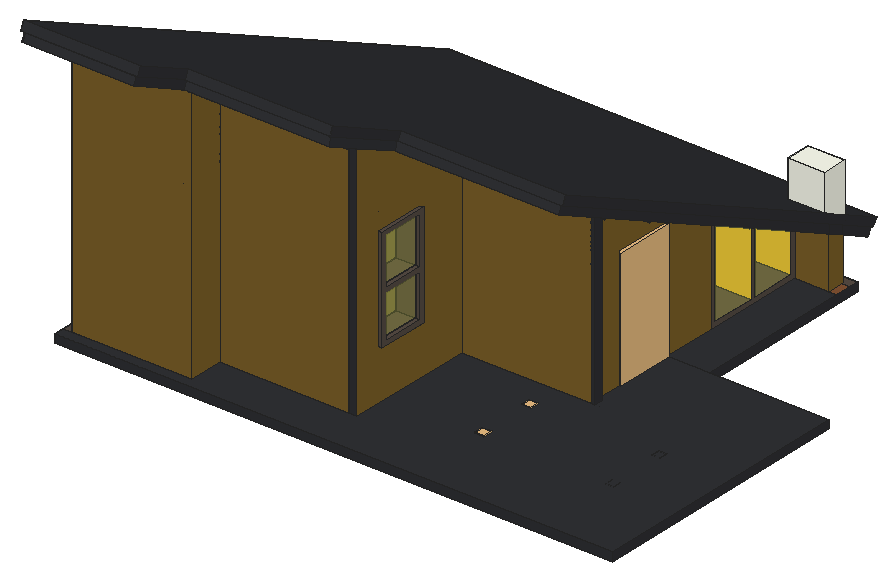
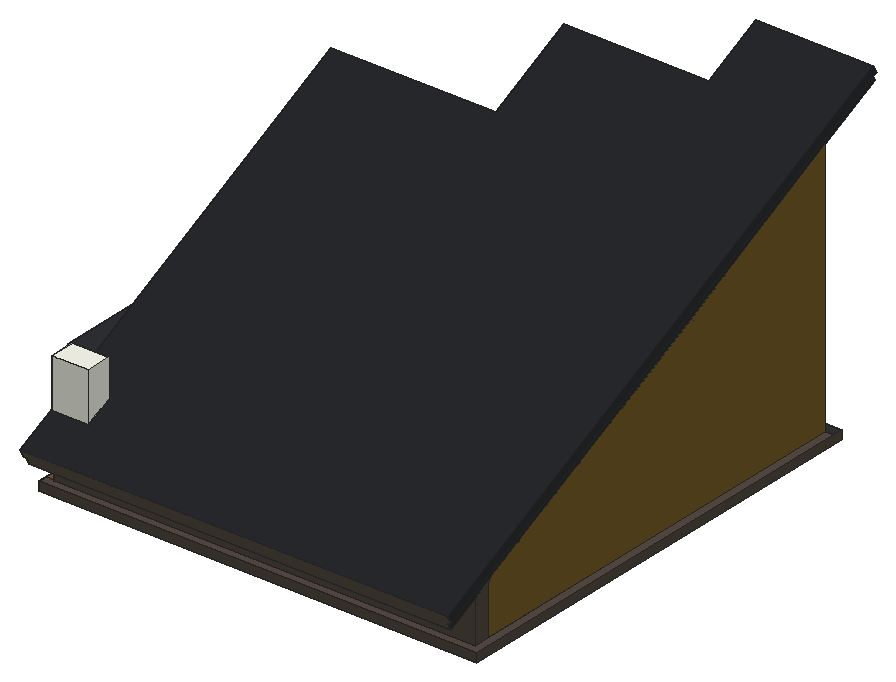
# SketchUp Ruby script. Lengths in inches.
U = 1.inch
M = Sketchup.active_model
def pt(a) = Geom::Point3d.new(a.map { |v| v * U })
def face(e, loops, mat)
  f = e.add_face(loops[0].map { |a| pt(a) })
  loops[1..].each { |l| e.add_face(l.map { |a| pt(a) }).erase! }
  f.material = f.back_material = mat if mat
  f
end
# faces: each face lists its corners as indices into pts; further lists are holes
def faces(e, pts, list, mat = nil) = list.each { |f| face(e, (f[0].is_a?(Array) ? f : [f]).map { |l| l.map { |i| pts[i] } }, mat) }
# xy, xz, yz: faces in a plane at the given z, y or x. An outline is a flat list of corners, or four numbers for a rectangle; further outlines are holes
def ring(l) = l.size == 4 ? [[l[0], l[1]], [l[2], l[1]], [l[2], l[3]], [l[0], l[3]]] : l.each_slice(2).to_a
def flat(e, list, mat, &to3) = list.each { |f| face(e, (f[0].is_a?(Array) ? f : [f]).map { |l| ring(l).map { |u, v| to3.(u, v) } }, mat) }
def xy(e, z, list, mat = nil) = flat(e, list, mat) { |x, y| [x, y, z] }
def xz(e, y, list, mat = nil) = flat(e, list, mat) { |x, z| [x, y, z] }
def yz(e, x, list, mat = nil) = flat(e, list, mat) { |y, z| [x, y, z] }
def lines(e, pts, list) = list.each { |a, b| e.add_line(pt(pts[a]), pt(pts[b])) }
# prism: a flat outline (further loops are holes) pulled along v
def prism(e, loops, v, mat = nil)
  f = face(e, loops, mat); d = Geom::Vector3d.new(v.map { |x| x * U })
  f.pushpull(f.normal.samedirection?(d) ? d.length : -d.length)
end
def box(e, o, s, mat = nil) = prism(e, [[o, [o[0] + s[0], o[1], o[2]], [o[0] + s[0], o[1] + s[1], o[2]], [o[0], o[1] + s[1], o[2]]]], [0, 0, s[2]], mat)
def at(x, y, z, deg = 0) = Geom::Transformation.translation(pt([x, y, z])) * Geom::Transformation.rotation(ORIGIN, Z_AXIS, deg.degrees)
def axes(o, x, y, z) = Geom::Transformation.new([*x, 0, *y, 0, *z, 0, *pt(o).to_a, 1])
def part(name) = M.definitions.add(name)
# library, detail: a bought-in or finely detailed component or shape, given as its bounding box
def library(name, o, s) = part(name).tap { |d| box(d.entities, o, s) }
def detail(e, o, s) = box(e.add_group.entities, o, s)
def put(e, d, t, mat = nil) = e.add_instance(d, t).tap { |i| i.material = mat if mat }
def group(e, t, mat = nil) = e.add_group.tap { |g| g.transformation = t; g.material = mat if mat }.entities
root = M.entities
M.materials.add("Asphalt_02_1K").color = [86, 76, 68]
M.materials.add("Concrete_04_1K").color = [254, 255, 241]
M.materials.add("D04_Dandelion_Burst").color = [255, 204, 50]
M.materials.add("Glass_Basic_01").color = [253, 255, 84]
M.materials["Glass_Basic_01"].alpha = 0.25
M.materials.add("Plywood_01_1K").color = [130, 82, 50]
M.materials.add("Plywood_01_1K1").color = [125, 97, 41]
M.materials.add("ThomThom - Buttons1").color = [48, 49, 53]
M.materials.add("ThomThom - Buttons2").color = [40, 40, 43]
c1 = library("Sphere Light\#2",[-3.27,-3.27,-3.27],[6.54,6.54,6.54])
c2 = library("Sphere Light\#3",[-3.12,-3.12,-3.12],[6.24,6.24,6.24])
c3 = library("Sphere Light",[-2.87,-2.87,-2.87],[5.74,5.74,5.74])
c4 = library("Sphere Light\#1",[-2.75,-2.75,-2.75],[5.5,5.5,5.5])
c5 = library("porta+4",[0.2,-5.42,1.33],[46.55,4.72,83.21])
c6 = library("Sphere Light\#4",[-2.75,-2.75,-2.75],[5.5,5.5,5.5])
c7 = library("Sphere Light\#5",[-3.11,-3.11,-3.11],[6.22,6.22,6.22])
c8 = library("Sphere Light\#6",[-2.79,-2.79,-2.79],[5.58,5.58,5.58])
c9 = library("Sphere Light\#7",[-3.09,-3.09,-3.09],[6.18,6.18,6.18])
c10 = library("Sphere Light\#8",[-2.99,-2.99,-2.99],[5.98,5.98,5.98])
xy(root,120,[[[24,80.18,24,398.18,330,398.18,330,269.18,413,269.18,413,80.18],[262.73,128.19,377,192.97],[377,116.19,389,128.19]],[[262.73,128.19,377,192.97],[274.73,137.19,275.51,137.29,276.23,137.59,276.85,138.07,277.33,138.69,277.63,139.42,277.73,140.19,362,140.19,362.1,139.42,362.4,138.69,362.88,138.07,363.5,137.59,364.22,137.29,365,137.19,365.78,137.29,366.5,137.59,367.12,138.07,367.6,138.69,367.9,139.42,368,140.19,367.9,140.97,367.6,141.69,367.12,142.3125,366.5,142.79,365.78,143.09,365,143.19,365,178,365.43,178,366.19,178.21,366.86,178.62,367.4,179.18,367.79,179.86,367.98,180.62,367.97,181.4,367.76,182.16,367.36,182.83,366.79,183.375,366.11,183.76,365.35,183.95,364.57,183.9375,363.81,183.73,363.14,183.33,362.6,182.76,362.21,182.08,362.02,181.32,362.03,180.97,277.73,180.97,277.63,181.75,277.33,182.47,276.85,183.09,276.23,183.57,275.51,183.87,274.73,183.97,273.96,183.87,273.23,183.57,272.61,183.09,272.14,182.47,271.84,181.75,271.73,180.97,271.84,180.19,272.14,179.47,272.61,178.85,273.23,178.37,273.96,178.07,274.73,177.97,274.73,143.19,273.96,143.09,273.23,142.79,272.61,142.3125,272.14,141.69,271.84,140.97,271.73,140.19,271.84,139.42,272.14,138.69,272.61,138.07,273.23,137.59,273.96,137.29]],[277.73,140.19,277.63,140.97,277.33,141.69,276.85,142.3125,276.23,142.79,275.51,143.09,274.73,143.19,274.73,177.97,275.51,178.07,276.23,178.37,276.85,178.85,277.33,179.47,277.63,180.19,277.73,180.97,362.03,180.97,362.03,180.54,362.24,179.79,362.64,179.11,363.21,178.57,363.89,178.18,364.65,177.99,365,178,365,143.19,364.22,143.09,363.5,142.79,362.88,142.3125,362.4,141.69,362.1,140.97,362,140.19]],"ThomThom - Buttons2")
xy(root,123,[[274.73,137.19,273.96,137.29,273.23,137.59,272.61,138.07,272.14,138.69,271.84,139.42,271.73,140.19,271.84,140.97,272.14,141.69,272.61,142.3125,273.23,142.79,273.96,143.09,274.73,143.19,275.51,143.09,276.23,142.79,276.85,142.3125,277.33,141.69,277.63,140.97,277.73,140.19,277.63,139.42,277.33,138.69,276.85,138.07,276.23,137.59,275.51,137.29],[365,137.19,364.22,137.29,363.5,137.59,362.88,138.07,362.4,138.69,362.1,139.42,362,140.19,362.1,140.97,362.4,141.69,362.88,142.3125,363.5,142.79,364.22,143.09,365,143.19,365.78,143.09,366.5,142.79,367.12,142.3125,367.6,141.69,367.9,140.97,368,140.19,367.9,139.42,367.6,138.69,367.12,138.07,366.5,137.59,365.78,137.29],[274.73,177.97,273.96,178.07,273.23,178.37,272.61,178.85,272.14,179.47,271.84,180.19,271.73,180.97,271.84,181.75,272.14,182.47,272.61,183.09,273.23,183.57,273.96,183.87,274.73,183.97,275.51,183.87,276.23,183.57,276.85,183.09,277.33,182.47,277.63,181.75,277.73,180.97,277.63,180.19,277.33,179.47,276.85,178.85,276.23,178.37,275.51,178.07],[364.65,177.99,363.89,178.18,363.21,178.57,362.64,179.11,362.24,179.79,362.03,180.54,362.03,180.97,362.02,181.32,362.21,182.08,362.6,182.76,363.14,183.33,363.81,183.73,364.57,183.9375,365.35,183.95,366.11,183.76,366.79,183.375,367.36,182.83,367.76,182.16,367.97,181.4,367.98,180.62,367.79,179.86,367.4,179.18,366.86,178.62,366.19,178.21,365.43,178,365,178]],"ThomThom - Buttons2")
xy(root,126,[[24,87.33,30,87.33,30,392.18,330,392.18,330,398.18,24,398.18],[36,93.33,108,93.33,108,136.18,196.36,136.18,196.36,202.18,36,202.18],[204,111.33,210,130.18],[114,117.33,204,130.18],[114,130.18,196.36,136.18],
  [196.36,130.18,204,136.18],[204,130.18,210,130.18,210,202.18,303,202.18,303,208.18,204,208.18,204,202.18,196.36,202.18,196.36,136.18,204,136.18],[30,202.18,36,380.18],[36,202.18,204,208.18],[36,208.18,108,380.18],
  [108,208.18,114,380.18],[114,208.18,204,380.18],[204,208.18,210,380.18],[210,208.18,294,380.18],[294,208.18,300,227.18],
  [294,269.18,300,380.18]],"Asphalt_02_1K")
xy(root,126,[[324,380.18,330,392.18]],"Plywood_01_1K")
xy(root,126,[[24,80.18,413,80.18,413,269.18,294,269.18,294,227.18,300,227.18,300,208.18,303,208.18,303,202.18,210,202.18,210,111.33,114,111.33,114,87.33,24,87.33],[300,269.18,330,380.18]],"ThomThom - Buttons1")
xy(root,129,[[267.06,311.18,300,342.68],[267.06,345.68,300,377.18]],"Asphalt_02_1K")
xy(root,162,[[210,129.33,213,165.33]],"Asphalt_02_1K")
xy(root,165,[[196.36,132.33,210,162.33],[210,132.33,213,162.33]],"Asphalt_02_1K")
xy(root,172.02,[[300,374.18,319.02,380.18],[319.02,374.18,324,380.18]],"Concrete_04_1K")
xy(root,195,[[196.36,132.33,210,162.33],[210,132.33,213,162.33]],"Asphalt_02_1K")
xy(root,198,[[196.36,132.33,210,162.33],[210,132.33,213,162.33]],"Asphalt_02_1K")
xy(root,203.52,[[300,374.18,325.7,392.18]],"Concrete_04_1K")
xy(root,210,[[294,227.18,300,269.18]],"Plywood_01_1K")
xy(root,231,[[196.36,132.33,210,162.33],[210,132.33,213,162.33]],"Asphalt_02_1K")
xy(root,234,[[210,129.33,213,165.33]],"Asphalt_02_1K")
xy(root,246,[[36,93.33,108,202.18],[108,130.18,114,136.18],[108,136.18,196.36,202.18],[196.36,136.18,204,202.18],[108,202.18,114,208.18],
  [114,202.18,196.36,208.18],[196.36,202.18,204,208.18],[204,202.18,210,208.18],[210,202.18,303,208.18]],"Asphalt_02_1K")
xy(root,290.37,[[114,111.33,204,117.33]],"Asphalt_02_1K")
xz(root,80.18,[[24,120,413,126]],"ThomThom - Buttons1")
xz(root,87.33,[[30,126,114,305.02]],"Plywood_01_1K1")
xz(root,93.33,[[36,126,108,246]],"Asphalt_02_1K")
xz(root,111.33,[[114,126,204,290.37]],"Plywood_01_1K1")
xz(root,111.33,[[204,126,210,293.3],[114,290.37,204,293.3]],"ThomThom - Buttons1")
xz(root,117.33,[[114,126,204,290.37]],"Asphalt_02_1K")
xz(root,129.33,[[210,162,213,234]],"Asphalt_02_1K")
xz(root,130.18,[[196.36,126,204,246],[196.36,246,204,284.09]],"Asphalt_02_1K")
xz(root,132.33,[[196.36,165,210,195],[210,165,213,195],[196.36,198,210,231],[210,198,213,231]],"Asphalt_02_1K")
xz(root,136.18,[[108,126,114,246]],"Asphalt_02_1K")
xz(root,162.33,[[196.36,165,210,195],[210,165,213,195],[196.36,198,210,231],[210,198,213,231]],"Asphalt_02_1K")
xz(root,165.33,[[210,162,213,234]],"Asphalt_02_1K")
xz(root,178,[[365,120,365.43,123]],"ThomThom - Buttons2")
xz(root,202.18,[[36,126,196.36,246],[196.36,126,204,246]],"Asphalt_02_1K")
xz(root,202.18,[[210,126,300,246]],"Plywood_01_1K1")
xz(root,202.18,[[300,126,303,246],[210,246,303,248.93]],"ThomThom - Buttons1")
xz(root,208.18,[[36,126,108,246],[108,126,114,246],[114,126,204,246],[204,126,210,246],[210,126,294,246],
  [294,126,300,246]],"Asphalt_02_1K")
xz(root,208.18,[[300,126,303,246]],"ThomThom - Buttons1")
xz(root,227.18,[[294,126,300,210]],"Plywood_01_1K")
xz(root,269.18,[[294,126,300,210]],"Plywood_01_1K")
xz(root,269.18,[[330,120,413,126]],"ThomThom - Buttons1")
xz(root,311.18,[[267.06,129,300,192.36]],"D04_Dandelion_Burst")
xz(root,342.68,[[267.06,129,300,176.98]],"D04_Dandelion_Burst")
xz(root,345.68,[[267.06,129,300,175.51]],"D04_Dandelion_Burst")
xz(root,374.18,[[300,178.28,325.7,203.52]],"Concrete_04_1K")
xz(root,377.18,[[267.06,129,300,160.125]],"D04_Dandelion_Burst")
xz(root,380.18,[[30,126,36,162],[36,126,108,162],[108,126,114,162],[114,126,204,162],[204,126,210,162],
  [210,126,294,162],[294,126,300,162],[300,162,324,172.02]],"Asphalt_02_1K")
xz(root,380.18,[[300,126,324,162]],"Plywood_01_1K1")
xz(root,392.18,[[30,126,324,156.14]],"Asphalt_02_1K")
xz(root,392.18,[[300,166.16,325.7,203.52]],"Concrete_04_1K")
xz(root,398.18,[[24,120,330,126]],"Asphalt_02_1K")
yz(root,24,[[80.18,120,398.18,126]],"Asphalt_02_1K")
yz(root,28,[[416.48,150.95,46.83,331.48,45.03,332.35,47.67,337.75,419.11,156.34]],"ThomThom - Buttons1")
yz(root,30,[[380.18,126,380.18,162,392.18,156.14,392.18,126]],"Asphalt_02_1K")
yz(root,30,[[87.33,126,87.33,305.02,208.18,246,380.18,162,380.18,126]],"Plywood_01_1K1")
yz(root,30,[[413.84,145.5625,392.18,156.14,380.18,162,208.18,246,87.33,305.02,44.2,326.09,46.83,331.48,416.48,150.95]],"ThomThom - Buttons1")
yz(root,36,[[93.33,126,202.18,246],[208.18,126,380.18,126,380.18,162,208.18,246]],"Asphalt_02_1K")
yz(root,108,[[93.33,126,116.18,246],[116.18,126,130.18,246],[130.18,126,136.18,246],[208.18,126,208.18,246,380.18,162,380.18,126]],"Asphalt_02_1K")
yz(root,108,[[87.33,305.02,89.96,310.41,80.27,315.15,46.83,331.48,44.2,326.09]],"ThomThom - Buttons1")
yz(root,110,[[85.96,312.37,88.59,317.76,47.67,337.75,45.03,332.35,80.27,315.15]],"ThomThom - Buttons1")
yz(root,114,[[117.33,126,130.18,246],[130.18,126,136.18,246],[208.18,126,380.18,126,380.18,162,208.18,246],[111.33,246,117.33,290.37],[117.33,246,130.18,246,130.18,284.09,117.33,290.37],
  [111.33,290.37,117.33,290.37,111.33,293.3]],"Asphalt_02_1K")
yz(root,114,[[87.33,126,111.33,126,111.33,293.3,87.33,305.02]],"Plywood_01_1K1")
yz(root,196.36,[[[130.18,126,202.18,246],[132.33,198,162.33,231],[132.33,165,162.33,195]],[130.18,246,130.18,284.09,208.18,246]],"Asphalt_02_1K")
yz(root,196.36,[[132.33,165,162.33,195],[132.33,198,162.33,231]],"Glass_Basic_01")
yz(root,204,[[111.33,126,117.33,290.37],[117.33,126,130.18,246],[202.18,126,208.18,246],[208.18,126,208.18,246,380.18,162,380.18,126],[111.33,290.37,111.33,293.3,117.33,290.37]],"Asphalt_02_1K")
yz(root,210,[[208.18,126,380.18,126,380.18,162,208.18,246],[202.18,246,208.18,246,202.18,248.93]],"Asphalt_02_1K")
yz(root,210,[[132.33,165,162.33,195],[132.33,198,162.33,231]],"Glass_Basic_01")
yz(root,210,[[[111.33,126,202.18,126,202.18,248.93,144.52,277.09,111.33,293.3],[129.33,162,165.33,234]]],"Plywood_01_1K1")
yz(root,210.9,[[145.36,283.36,147.99,288.75,88.59,317.76,85.96,312.37]],"ThomThom - Buttons1")
yz(root,213,[[[129.33,162,165.33,234],[132.33,198,162.33,231],[132.33,165,162.33,195]]],"Asphalt_02_1K")
yz(root,267.06,[[311.18,129,342.68,129,342.68,176.98,311.18,192.36],[345.68,129,377.18,129,377.18,160.125,345.68,175.51]],"D04_Dandelion_Burst")
yz(root,294,[[227.18,126,269.18,210]],"Plywood_01_1K")
yz(root,300,[[[308.18,126,380.18,126,380.18,162,308.18,197.16],[311.18,129,311.18,192.36,342.68,176.98,342.68,129],[345.68,129,345.68,175.51,377.18,160.125,377.18,129]],[392.18,156.14,392.18,162,380.18,162]],"Asphalt_02_1K")
yz(root,300,[[392.18,166.16,380.18,172.02,381.5,174.71,392.18,169.49],[392.18,169.49,381.5,174.71,380.18,172.02,374.18,172.02,374.18,203.52,392.18,203.52]],"Concrete_04_1K")
yz(root,300,[[311.18,129,342.68,129,342.68,176.98,311.18,192.36],[345.68,129,377.18,129,377.18,160.125,345.68,175.51]],"Glass_Basic_01")
yz(root,300,[[208.18,126,227.18,126,227.18,210,269.18,210,269.18,126,308.18,126,308.18,197.16,208.18,246]],"Plywood_01_1K1")
yz(root,303,[[202.18,126,208.18,246],[202.18,246,208.18,246,202.18,248.93]],"ThomThom - Buttons1")
yz(root,324,[[380.18,126,392.18,126,392.18,156.14,380.18,162]],"Plywood_01_1K1")
yz(root,324,[[413.84,145.5625,416.48,150.95,392.18,162.82,392.18,156.14],[392.18,156.14,392.18,162.82,380.18,168.68,380.18,162],[380.18,162,380.18,168.68,147.15,282.48,144.52,277.09]],"ThomThom - Buttons1")
yz(root,325.7,[[392.18,166.16,392.18,203.52,374.18,203.52,374.18,178.28,375.5,177.64,381.5,174.71,380.18,172.02]],"Concrete_04_1K")
yz(root,326,[[416.48,150.95,419.11,156.34,381.5,174.71,375.5,177.64,374.18,178.28,147.99,288.75,145.36,283.36]],"ThomThom - Buttons1")
yz(root,330,[[269.18,120,398.18,126]],"ThomThom - Buttons1")
yz(root,362.03,[[180.54,120,180.97,123]],"ThomThom - Buttons2")
yz(root,413,[[80.18,120,269.18,126]],"ThomThom - Buttons1")
p = [[305.66,263.57,36.875],[305.66,233.28,36.875],[305.71,233.28,31.86],[305.71,263.57,31.86],[305.33,263.57,66.67],[305.33,233.28,66.67],
  [305.4,233.28,59.8],[305.4,263.57,59.8],[274.73,137.19,120],[273.96,137.29,120],[273.96,137.29,123],[274.73,137.19,123],
  [275.51,137.29,120],[275.51,137.29,123],[365,137.19,120],[364.22,137.29,120],[364.22,137.29,123],[365,137.19,123],
  [365.78,137.29,120],[365.78,137.29,123],[273.23,137.59,120],[273.23,137.59,123],[276.23,137.59,120],[276.23,137.59,123],
  [363.5,137.59,120],[363.5,137.59,123],[366.5,137.59,120],[366.5,137.59,123],[272.61,138.07,120],[272.61,138.07,123],
  [276.85,138.07,120],[276.85,138.07,123],[362.88,138.07,120],[362.88,138.07,123],[367.12,138.07,120],[367.12,138.07,123],
  [272.14,138.69,120],[272.14,138.69,123],[277.33,138.69,120],[277.33,138.69,123],[362.4,138.69,120],[362.4,138.69,123],
  [367.6,138.69,120],[367.6,138.69,123],[271.84,139.42,120],[271.84,139.42,123],[277.63,139.42,120],[277.63,139.42,123],
  [362.1,139.42,120],[362.1,139.42,123],[367.9,139.42,120],[367.9,139.42,123],[271.73,140.19,120],[271.73,140.19,123],
  [277.73,140.19,120],[277.73,140.19,123],[362,140.19,120],[362,140.19,123],[368,140.19,120],[368,140.19,123],
  [271.84,140.97,120],[271.84,140.97,123],[277.63,140.97,120],[277.63,140.97,123],[362.1,140.97,120],[362.1,140.97,123],
  [367.9,140.97,120],[367.9,140.97,123],[272.14,141.69,120],[272.14,141.69,123],[277.33,141.69,120],[277.33,141.69,123],
  [362.4,141.69,120],[362.4,141.69,123],[367.6,141.69,120],[367.6,141.69,123],[272.61,142.3125,120],[272.61,142.3125,123],
  [276.85,142.3125,120],[276.85,142.3125,123],[362.88,142.3125,120],[362.88,142.3125,123],[367.12,142.3125,120],[367.12,142.3125,123],
  [273.23,142.79,120],[273.23,142.79,123],[276.23,142.79,120],[276.23,142.79,123],[363.5,142.79,120],[363.5,142.79,123],
  [366.5,142.79,120],[366.5,142.79,123],[273.96,143.09,120],[273.96,143.09,123],[275.51,143.09,120],[275.51,143.09,123],
  [364.22,143.09,120],[364.22,143.09,123],[365.78,143.09,120],[365.78,143.09,123],[274.73,143.19,120],[274.73,143.19,123],
  [365,143.19,120],[365,143.19,123],[274.73,177.97,120],[273.96,178.07,120],[273.96,178.07,123],[274.73,177.97,123],
  [275.51,178.07,120],[275.51,178.07,123],[364.65,177.99,120],[363.89,178.18,120],[363.89,178.18,123],[364.65,177.99,123],
  [365,178,120],[365,178,123],[366.19,178.21,120],[365.43,178,120],[365.43,178,123],[366.19,178.21,123],
  [273.23,178.37,120],[273.23,178.37,123],[276.23,178.37,120],[276.23,178.37,123],[363.21,178.57,120],[363.21,178.57,123],
  [366.86,178.62,120],[366.86,178.62,123],[272.61,178.85,120],[272.61,178.85,123],[276.85,178.85,120],[276.85,178.85,123],
  [362.64,179.11,120],[362.64,179.11,123],[367.4,179.18,120],[367.4,179.18,123],[272.14,179.47,120],[272.14,179.47,123],
  [277.33,179.47,120],[277.33,179.47,123],[362.24,179.79,120],[362.24,179.79,123],[367.79,179.86,120],[367.79,179.86,123],
  [271.84,180.19,120],[271.84,180.19,123],[277.63,180.19,120],[277.63,180.19,123],[362.03,180.54,120],[362.03,180.54,123],
  [367.98,180.62,120],[367.98,180.62,123],[271.73,180.97,120],[271.73,180.97,123],[277.73,180.97,120],[277.73,180.97,123],
  [367.97,181.4,120],[367.97,181.4,123],[271.84,181.75,120],[271.84,181.75,123],[277.63,181.75,120],[277.63,181.75,123],
  [362.03,180.97,120],[362.02,181.32,120],[362.02,181.32,123],[362.03,180.97,123],[362.21,182.08,120],[362.21,182.08,123],
  [367.76,182.16,120],[367.76,182.16,123],[272.14,182.47,120],[272.14,182.47,123],[277.33,182.47,120],[277.33,182.47,123],
  [362.6,182.76,120],[362.6,182.76,123],[367.36,182.83,120],[367.36,182.83,123],[272.61,183.09,120],[272.61,183.09,123],
  [276.85,183.09,120],[276.85,183.09,123],[363.14,183.33,120],[363.14,183.33,123],[366.79,183.375,120],[366.79,183.375,123],
  [273.23,183.57,120],[273.23,183.57,123],[276.23,183.57,120],[276.23,183.57,123],[363.81,183.73,120],[363.81,183.73,123],
  [366.11,183.76,120],[366.11,183.76,123],[273.96,183.87,120],[273.96,183.87,123],[275.51,183.87,120],[275.51,183.87,123],
  [364.57,183.9375,120],[364.57,183.9375,123],[365.35,183.95,120],[365.35,183.95,123],[274.73,183.97,120],[274.73,183.97,123],
  [30,413.84,145.5625],[324,413.84,145.5625],[324,392.18,156.14],[300,392.18,156.14],[294,392.18,156.14],[210,392.18,156.14],
  [204,392.18,156.14],[114,392.18,156.14],[108,392.18,156.14],[36,392.18,156.14],[30,392.18,156.14],[324,416.48,150.95],
  [30,416.48,150.95],[28,416.48,150.95],[28,419.11,156.34],[326,419.11,156.34],[326,416.48,150.95],[299.65,266,157.55],
  [299.65,230.78,157.55],[299.73,230.78,150.125],[299.73,266,150.125],[30,46.83,331.48],[28,46.83,331.48],[324,147.15,282.48],
  [324,380.18,168.68],[324,392.18,162.82],[326,145.36,283.36],[324,145.36,283.36],[30,380.18,162],[36,380.18,162],
  [108,380.18,162],[114,380.18,162],[204,380.18,162],[210,380.18,162],[294,380.18,162],[300,380.18,162],
  [324,380.18,162],[325.7,375.5,177.64],[325.7,381.5,174.71],[326,381.5,174.71],[28,47.67,337.75],[110,47.67,337.75],
  [110,88.59,317.76],[210.9,88.59,317.76],[210.9,147.99,288.75],[326,147.99,288.75],[326,374.18,178.28],[325.7,374.18,178.28],
  [300,377.18,160.125],[300,345.68,175.51],[267.06,345.68,175.51],[267.06,377.18,160.125],[300,308.18,197.16],[324,144.52,277.09],
  [210,144.52,277.09],[210,202.18,248.93],[303,202.18,248.93],[303,208.18,246],[300,208.18,246],[313.75,361.64,171.06],
  [312.98,361.75,171],[312.2,361.67,171.04],[311.47,361.42,171.16],[310.84,361,171.37],[310.34,360.46,171.63],[310.03,359.8125,171.95],
  [309.91,359.12,172.29],[309.99,358.42,172.63],[310.27,357.76,172.95],[310.73,357.19,173.23],[311.34,356.75,173.44],[312.06,356.47,173.58],
  [312.83,356.36,173.64],[313.61,356.43,173.6],[314.34,356.69,173.48],[314.97,357.1,173.27],[315.47,357.65,173.01],[315.78,358.29,172.69],
  [315.9,358.99,172.35],[315.82,359.6875,172.01],[315.54,360.34,171.6875],[315.08,360.91,171.41],[314.47,361.35,171.2],[316.81,283.77,209.08],
  [316.72,284.47,208.74],[316.44,285.13,208.42],[315.98,285.7,208.14],[315.37,286.14,207.93],[314.65,286.43,207.79],[313.88,286.53,207.74],
  [313.1,286.46,207.77],[312.37,286.21,207.9],[311.74,285.79,208.1],[311.25,285.24,208.37],[310.93,284.6,208.68],[310.81,283.91,209.02],
  [310.89,283.21,209.36],[311.17,282.55,209.68],[311.63,281.98,209.96],[312.24,281.54,210.18],[312.96,281.25,210.3125],[313.73,281.14,210.37],
  [314.51,281.22,210.33],[315.24,281.47,210.21],[315.875,281.89,210],[316.37,282.43,209.74],[316.68,283.08,209.42],[317.94,233.4,233.6875],
  [317.86,234.1,233.34],[317.58,234.75,233.02],[317.12,235.32,232.75],[316.51,235.76,232.53],[315.79,236.05,232.39],[315.02,236.16,232.34],
  [314.24,236.08,232.375],[313.51,235.83,232.5],[312.875,235.42,232.7],[312.38,234.87,232.97],[312.07,234.23,233.28],[311.95,233.53,233.62],
  [312.03,232.83,233.96],[312.3125,232.17,234.28],[312.77,231.6,234.5625],[313.38,231.16,234.78],[314.1,230.88,234.92],[314.87,230.77,234.97],
  [315.65,230.84,234.93],[316.38,231.1,234.81],[317.01,231.51,234.61],[317.51,232.06,234.34],[317.82,232.7,234.03],[318.57,194.02,252.92],
  [318.49,194.72,252.57],[318.21,195.38,252.25],[317.74,195.95,251.98],[317.13,196.39,251.76],[316.42,196.67,251.62],[315.64,196.78,251.57],
  [314.87,196.71,251.6],[314.14,196.46,251.73],[313.5,196.04,251.93],[313.01,195.49,252.2],[312.69,194.85,252.51],[312.57,194.15,252.85],
  [312.66,193.45,253.19],[312.9375,192.8,253.51],[313.4,192.23,253.79],[314.01,191.79,254.01],[314.72,191.5,254.15],[315.5,191.39,254.2],
  [316.28,191.47,254.16],[317.01,191.72,254.04],[317.64,192.14,253.84],[318.13,192.68,253.57],[318.45,193.33,253.26],[316.37,323.08,189.89],
  [316.29,323.78,189.55],[316.01,324.44,189.23],[315.55,325,188.95],[314.9375,325.45,188.73],[314.22,325.73,188.59],[313.45,325.84,188.54],
  [312.67,325.77,188.58],[311.9375,325.51,188.7],[311.3,325.1,188.9],[310.8125,324.55,189.17],[310.5,323.91,189.48],[310.375,323.21,189.82],
  [310.46,322.51,190.17],[310.74,321.85,190.49],[311.2,321.29,190.76],[311.8125,320.84,190.98],[312.53,320.56,191.12],[313.3,320.45,191.17],
  [314.08,320.53,191.14],[314.81,320.78,191.01],[315.44,321.19,190.81],[315.93,321.74,190.54],[316.25,322.38,190.23],[30,208.18,246],
  [36,208.18,246],[108,208.18,246],[114,208.18,246],[204,208.18,246],[196.36,208.18,246],[210,208.18,246],
  [294,208.18,246],[324,380.18,172.02],[325.7,380.18,172.02],[325.7,392.18,166.16],[324,392.18,166.16],[300,392.18,166.16],
  [300,380.18,172.02],[319.02,380.18,172.02],[312.2,362.55,172.84],[311.47,362.3,172.96],[313.75,362.52,172.85],[312.98,362.625,172.8],
  [314.47,362.23,172.99],[315.08,361.79,173.21],[310.84,361.88,173.16],[315.54,361.22,173.49],[310.34,361.33,173.43],[310.03,360.69,173.74],
  [315.82,360.5625,173.81],[309.91,360,174.08],[315.9,359.86,174.15],[300,381.5,174.71],[319.02,381.5,174.71],[324,381.5,174.71],
  [309.99,359.3,174.43],[315.78,359.17,174.49],[310.27,358.64,174.75],[315.47,358.53,174.8],[299.37,266,182.76],[299.37,230.78,182.76],
  [299.48,230.78,172.83],[299.48,266,172.83],[314.97,357.98,175.07],[314.34,357.5625,175.27],[313.61,357.31,175.4],[312.83,357.24,175.43],
  [312.06,357.34,175.38],[311.34,357.63,175.24],[310.73,358.07,175.02],[326,375.5,177.64],[300,342.68,176.98],[300,311.18,192.36],
  [267.06,311.18,192.36],[267.06,342.68,176.98],[314.22,326.61,190.39],[313.45,326.72,190.34],[312.67,326.64,190.375],[314.9375,326.32,190.53],
  [311.9375,326.39,190.5],[315.55,325.88,190.74],[311.3,325.98,190.7],[316.01,325.3125,191.02],[310.8125,325.43,190.97],[316.29,324.66,191.34],
  [310.5,324.78,191.28],[316.37,323.96,191.69],[310.375,324.09,191.62],[310.46,323.39,191.96],[316.25,323.26,192.02],[315.93,322.62,192.34],
  [310.74,322.73,192.28],[315.44,322.07,192.61],[314.81,321.66,192.81],[314.08,321.4,192.93],[313.3,321.33,192.97],[312.53,321.4375,192.92],
  [311.8125,321.72,192.78],[311.2,322.16,192.5625],[314.65,287.3,209.59],[313.88,287.41,209.53],[313.1,287.34,209.57],[315.37,287.02,209.72],
  [312.37,287.08,209.69],[315.98,286.58,209.94],[311.74,286.67,209.9],[316.44,286.01,210.22],[311.25,286.12,210.16],[316.72,285.35,210.54],
  [310.93,285.48,210.48],[316.81,284.65,210.88],[310.81,284.78,210.82],[310.89,284.08,211.16],[316.68,283.96,211.22],[316.37,283.3125,211.53],
  [311.17,283.43,211.48],[315.875,282.77,211.8],[315.24,282.35,212],[314.51,282.1,212.13],[313.73,282.02,212.16],[312.96,282.13,212.11],
  [312.24,282.42,211.97],[311.63,282.86,211.76],[315.79,236.93,234.1875],[315.02,237.04,234.13],[314.24,236.96,234.17],[313.51,236.71,234.29],
  [316.51,236.64,234.33],[317.12,236.2,234.54],[312.875,236.29,234.5],[317.58,235.63,234.82],[312.38,235.75,234.76],[317.86,234.98,235.14],
  [312.07,235.1,235.08],[317.94,234.28,235.48],[311.95,234.41,235.42],[312.03,233.71,235.76],[317.82,233.58,235.82],[317.51,232.9375,236.14],
  [312.3125,233.05,236.08],[317.01,232.39,236.4],[316.38,231.97,236.61],[315.65,231.72,236.73],[314.87,231.65,236.77],[314.1,231.76,236.71],
  [313.38,232.04,236.57],[312.77,232.48,236.36],[30,87.33,305.02],[36,87.33,305.02],[108,87.33,305.02],[114,87.33,305.02],
  [114,111.33,293.3],[114,117.33,290.37],[114,130.18,284.09],[210,111.33,293.3],[204,111.33,293.3],[204,117.33,290.37],
  [204,130.18,284.09],[196.36,130.18,284.09],[317.13,197.27,253.56],[316.42,197.55,253.42],[314.87,197.59,253.4],[314.14,197.33,253.52],
  [315.64,197.66,253.36],[313.5,196.92,253.73],[317.74,196.83,253.77],[313.01,196.37,253.99],[318.21,196.26,254.05],[312.69,195.73,254.31],
  [318.49,195.6,254.37],[312.57,195.03,254.65],[318.57,194.9,254.71],[318.45,194.2,255.05],[312.66,194.33,254.99],[312.9375,193.68,255.3125],
  [318.13,193.5625,255.37],[317.64,193.01,255.63],[317.01,192.6,255.84],[316.28,192.35,255.96],[315.5,192.27,256],[314.72,192.38,255.94],
  [314.01,192.67,255.8],[313.4,193.11,255.59],[208.9,145.36,283.36],[208.9,89.96,310.41],[210,87.33,305.02],[208.9,147.15,282.48],
  [210.9,145.36,283.36],[210.9,85.96,312.37],[208.9,85.96,312.37],[108,44.2,326.09],[30,44.2,326.09],[108,89.96,310.41],
  [110,85.96,312.37],[110,80.27,315.15],[108,80.27,315.15],[108,46.83,331.48],[110,45.03,332.35],[108,45.03,332.35],
  [28,45.03,332.35],[306,202.18,120],[306,202.18,126],[306,230.18,90],[306,266.18,90],[306,230.18,87],
  [306,266.18,87],[300,392.18,162],[30,392.18,162],[210,130.18,246],[204,130.18,246],[36,202.18,246],
  [30,202.18,246],[108,93.33,246],[108,87.33,246],[324,381.59,171.33],[326,380.18,172.02],[326,374.18,172.02],
  [324,374.18,172.02],[326,374.18,174.95],[300,374.18,174.95],[300,393.5,168.85],[326,392.18,166.16]]
faces(root,p,[[0,1,2,3],[4,5,6,7],[221,222,223,224],[418,419,420,421]],"Glass_Basic_01")
faces(root,p,[[8,9,10,11],[12,8,11,13],[14,15,16,17],[18,14,17,19],[9,20,21,10],[22,12,13,23],[15,24,25,16],[26,18,19,27],
  [20,28,29,21],[30,22,23,31],[24,32,33,25],[34,26,27,35],[28,36,37,29],[38,30,31,39],[32,40,41,33],[42,34,35,43],
  [36,44,45,37],[46,38,39,47],[40,48,49,41],[50,42,43,51],[44,52,53,45],[54,46,47,55],[48,56,57,49],[58,50,51,59],
  [52,60,61,53],[62,54,55,63],[56,64,65,57],[66,58,59,67],[60,68,69,61],[70,62,63,71],[64,72,73,65],[74,66,67,75],
  [68,76,77,69],[78,70,71,79],[72,80,81,73],[82,74,75,83],[76,84,85,77],[86,78,79,87],[80,88,89,81],[90,82,83,91],
  [84,92,93,85],[94,86,87,95],[88,96,97,89],[98,90,91,99],[92,100,101,93],[100,94,95,101],[96,102,103,97],[102,98,99,103],
  [104,105,106,107],[108,104,107,109],[110,111,112,113],[114,110,113,115],[116,117,118,119],[105,120,121,106],[122,108,109,123],[111,124,125,112],
  [126,116,119,127],[120,128,129,121],[130,122,123,131],[124,132,133,125],[134,126,127,135],[128,136,137,129],[138,130,131,139],[132,140,141,133],
  [142,134,135,143],[136,144,145,137],[146,138,139,147],[140,148,149,141],[150,142,143,151],[144,152,153,145],[154,146,147,155],[156,150,151,157],
  [152,158,159,153],[160,154,155,161],[162,163,164,165],[163,166,167,164],[168,156,157,169],[158,170,171,159],[172,160,161,173],[166,174,175,167],
  [176,168,169,177],[170,178,179,171],[180,172,173,181],[174,182,183,175],[184,176,177,185],[178,186,187,179],[188,180,181,189],[182,190,191,183],
  [192,184,185,193],[186,194,195,187],[196,188,189,197],[190,198,199,191],[200,192,193,201],[194,202,203,195],[202,196,197,203],[198,200,201,199]],"ThomThom - Buttons2")
faces(root,p,[[204,205,206,207,208,209,210,211,212,213,214],[215,205,204,216,217,218,219,220],[216,225,226,217],[227,228,229,215,220,230,231],[232,214,213,233],[233,213,212,234],[234,212,211,235],[235,211,210,236],
  [236,210,209,237],[237,209,208,238],[238,208,207,239],[239,207,206,240],[383,232,233,384],[233,234,385,384],[386,235,234,385],[387,388,386,235,236],
  [387,236,237,389],[390,238,239,256,262],[383,506,507,384],[385,508,507,384],[385,508,509,510,511,512,386],[258,513,514,515,516,517,388,387,389,259],[516,515,511,512,386,388,517],[390,262,261,260,259,389],
  [545,227,231,546,542],[543,542,546,547,548],[515,514,510,511],[551,543,548,552,553,554],[555,554,553,556,557],[225,555,557,558,226]],"Asphalt_02_1K")
faces(root,p,[[241,242,243,219,218,244,245,246,247,248,249,250,251],[[256,239,240,257,258,259,260,261,262],[263,264,265,266,267,268,269,270,271,272,273,274,275,276,277,278,279,280,281,282,283,284,285,286],[287,288,289,290,291,292,293,294,295,296,297,298,299,300,301,302,303,304,305,306,307,308,309,310],[311,312,313,314,315,316,317,318,319,320,321,322,323,324,325,326,327,328,329,330,331,332,333,334],[335,336,337,338,339,340,341,342,343,344,345,346,347,348,349,350,351,352,353,354,355,356,357,358],[359,360,361,362,363,364,365,366,367,368,369,370,371,372,373,374,375,376,377,378,379,380,381,382]],[391,392,393,394,395,396,397],[266,265,398,399],[264,263,400,401],[265,264,401,398],[263,286,402,400],[286,285,403,402],
  [267,266,399,404],[285,284,405,403],[268,267,404,406],[269,268,406,407],[284,283,408,405],[270,269,407,409],[283,282,410,408],[397,396,411,412],
  [391,397,412,413],[413,242,392,391],[271,270,409,414],[282,281,415,410],[272,271,414,416],[281,280,417,415],[401,400,402,403,405,408,410,415,417,422,423,424,425,426,427,428,416,414,409,407,406,404,399,398],[273,272,416,428],
  [280,279,422,417],[274,273,428,427],[279,278,423,422],[275,274,427,426],[278,277,424,423],[276,275,426,425],[277,276,425,424],[429,241,251,250],
  [365,364,434,435],[366,365,435,436],[364,363,437,434],[367,366,436,438],[363,362,439,437],[368,367,438,440],[362,361,441,439],[369,368,440,442],
  [361,360,443,441],[370,369,442,444],[360,359,445,443],[371,370,444,446],[372,371,446,447],[359,382,448,445],[382,381,449,448],[373,372,447,450],
  [435,434,437,439,441,443,445,448,449,451,452,453,454,455,456,457,450,447,446,444,442,440,438,436],[381,380,451,449],[374,373,450,457],[375,374,457,456],[380,379,452,451],[379,378,453,452],[376,375,456,455],[377,376,455,454],
  [378,377,454,453],[293,292,458,459],[294,293,459,460],[292,291,461,458],[295,294,460,462],[291,290,463,461],[296,295,462,464],[290,289,465,463],
  [297,296,464,466],[289,288,467,465],[298,297,466,468],[288,287,469,467],[299,298,468,470],[300,299,470,471],[287,310,472,469],[310,309,473,472],
  [301,300,471,474],[459,458,461,463,465,467,469,472,473,475,476,477,478,479,480,481,474,471,470,468,466,464,462,460],[309,308,475,473],[302,301,474,481],[303,302,481,480],[308,307,476,475],[307,306,477,476],[304,303,480,479],
  [305,304,479,478],[306,305,478,477],[317,316,482,483],[318,317,483,484],[319,318,484,485],[316,315,486,482],[315,314,487,486],[320,319,485,488],
  [314,313,489,487],[321,320,488,490],[313,312,491,489],[322,321,490,492],[312,311,493,491],[323,322,492,494],[324,323,494,495],[311,334,496,493],
  [334,333,497,496],[325,324,495,498],[483,482,486,487,489,491,493,496,497,499,500,501,502,503,504,505,498,495,494,492,490,488,485,484],[333,332,499,497],[326,325,498,505],[332,331,500,499],[327,326,505,504],[331,330,501,500],
  [328,327,504,503],[329,328,503,502],[330,329,502,501],[340,339,518,519],[343,342,520,521],[342,341,522,520],[341,340,519,522],[344,343,521,523],
  [339,338,524,518],[345,344,523,525],[338,337,526,524],[346,345,525,527],[337,336,528,526],[347,346,527,529],[336,335,530,528],[335,358,531,530],
  [348,347,529,532],[349,348,532,533],[358,357,534,531],[522,519,518,524,526,528,530,531,534,535,536,537,538,539,540,541,533,532,529,527,525,523,521,520],[350,349,533,541],[357,356,535,534],[356,355,536,535],[351,350,541,540],
  [352,351,540,539],[355,354,537,536],[353,352,539,538],[354,353,538,537],[542,543,544,513,258,545],[257,227,545,258],[230,249,248,546,231],[544,509,510,514,513],
  [507,508,549,550,506],[544,543,551,508,509],[547,247,246,552,548],[549,555,225,550],[556,245,244,558,557]],"ThomThom - Buttons1")
faces(root,p,[[252,253,254,255],[430,431,432,433]],"D04_Dandelion_Burst")
faces(root,p,[[429,243,242,241]],"Concrete_04_1K")
lines(root,p,[[559,560],[561,562],[563,564],[565,566],[567,568],[569,570],[387,516],[571,572],[391,573],[229,394],[574,392],[575,576],
  [577,578],[395,579],[580,393]])
put(root,c1,at(274.66,140.45,123),"Asphalt_02_1K")
put(root,c2,at(274.89,181.11,123),"Asphalt_02_1K")
put(root,c3,at(365.1,140.36,123),"Asphalt_02_1K")
put(root,c4,at(364.9,181.2,123),"Asphalt_02_1K")
put(root,c5,axes([301.84,269.36,124.63],[0,-0.90228,0],[1,0,0],[0,0,0.99642]),"Asphalt_02_1K")
put(root,c6,at(312.7,360.09,174.04),"Asphalt_02_1K")
put(root,c7,at(313.16,323.86,191.73),"Asphalt_02_1K")
put(root,c8,at(313.74,284.72,210.85),"Asphalt_02_1K")
put(root,c9,at(314.84,234.37,235.4375),"Asphalt_02_1K")
put(root,c10,at(315.58,194.97,254.68),"Asphalt_02_1K")
